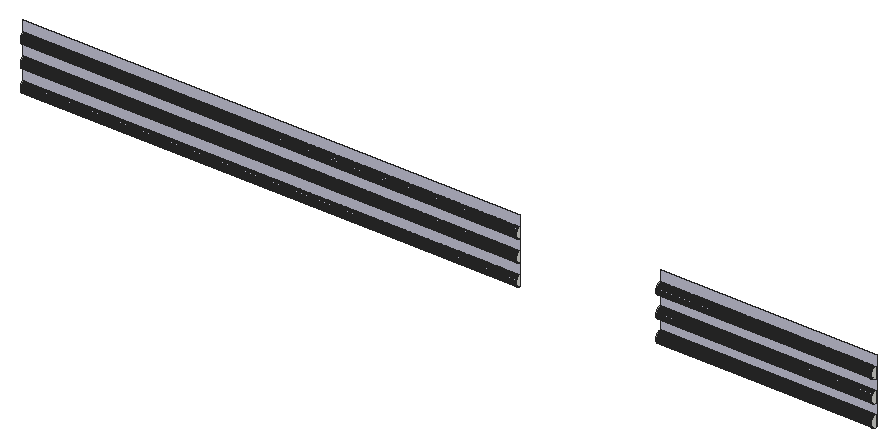
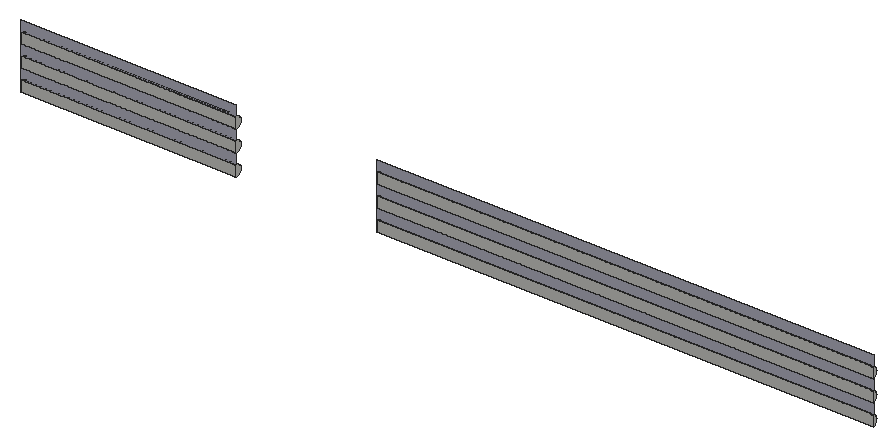
# SketchUp Ruby script. Lengths in millimetres.
U = 1.mm
M = Sketchup.active_model
def pt(a) = Geom::Point3d.new(a.map { |v| v * U })
def face(e, loops, mat)
  f = e.add_face(loops[0].map { |a| pt(a) })
  loops[1..].each { |l| e.add_face(l.map { |a| pt(a) }).erase! }
  f.material = f.back_material = mat if mat
  f
end
# faces: each face lists its corners as indices into pts; further lists are holes
def faces(e, pts, list, mat = nil) = list.each { |f| face(e, (f[0].is_a?(Array) ? f : [f]).map { |l| l.map { |i| pts[i] } }, mat) }
# xy, xz, yz: faces in a plane at the given z, y or x. An outline is a flat list of corners, or four numbers for a rectangle; further outlines are holes
def ring(l) = l.size == 4 ? [[l[0], l[1]], [l[2], l[1]], [l[2], l[3]], [l[0], l[3]]] : l.each_slice(2).to_a
def flat(e, list, mat, &to3) = list.each { |f| face(e, (f[0].is_a?(Array) ? f : [f]).map { |l| ring(l).map { |u, v| to3.(u, v) } }, mat) }
def xy(e, z, list, mat = nil) = flat(e, list, mat) { |x, y| [x, y, z] }
def xz(e, y, list, mat = nil) = flat(e, list, mat) { |x, z| [x, y, z] }
def yz(e, x, list, mat = nil) = flat(e, list, mat) { |y, z| [x, y, z] }
def lines(e, pts, list) = list.each { |a, b| e.add_line(pt(pts[a]), pt(pts[b])) }
# prism: a flat outline (further loops are holes) pulled along v
def prism(e, loops, v, mat = nil)
  f = face(e, loops, mat); d = Geom::Vector3d.new(v.map { |x| x * U })
  f.pushpull(f.normal.samedirection?(d) ? d.length : -d.length)
end
def box(e, o, s, mat = nil) = prism(e, [[o, [o[0] + s[0], o[1], o[2]], [o[0] + s[0], o[1] + s[1], o[2]], [o[0], o[1] + s[1], o[2]]]], [0, 0, s[2]], mat)
def at(x, y, z, deg = 0) = Geom::Transformation.translation(pt([x, y, z])) * Geom::Transformation.rotation(ORIGIN, Z_AXIS, deg.degrees)
def axes(o, x, y, z) = Geom::Transformation.new([*x, 0, *y, 0, *z, 0, *pt(o).to_a, 1])
def part(name) = M.definitions.add(name)
# library, detail: a bought-in or finely detailed component or shape, given as its bounding box
def library(name, o, s) = part(name).tap { |d| box(d.entities, o, s) }
def detail(e, o, s) = box(e.add_group.entities, o, s)
def put(e, d, t, mat = nil) = e.add_instance(d, t).tap { |i| i.material = mat if mat }
def group(e, t, mat = nil) = e.add_group.tap { |g| g.transformation = t; g.material = mat if mat }.entities
root = M.entities
M.materials.add("[0116_Lavender]").color = [197, 197, 214]
xz(root,16548.1,[[11038.5,5045.1,25059.3,5349.9],[29021.7,5045.1,35117.7,5349.9],[11038.5,5654.7,25059.3,5959.5],[29021.7,5654.7,35117.7,5959.5],[11038.5,6264.3,25059.3,6569.1],
  [29021.7,6264.3,35117.7,6569.1]])
xz(root,16548.1,[[11038.5,5349.9,25059.3,5654.7],[29021.7,5349.9,35117.7,5654.7],[11038.5,5959.5,25059.3,6264.3],[29021.7,5959.5,35117.7,6264.3],[11038.5,6569.1,25059.3,6873.9],
  [29021.7,6569.1,35117.7,6873.9]],"[0116_Lavender]")
yz(root,11038.5,[[16548.1,5045.1,16536.2,5050.4,16524.8,5056.7,16514,5063.8,16503.7,5071.8,16494.1,5080.6,16485.2,5090.1,16477.1,5100.2,16469.8,5111,16463.4,5122.3,16458,5134.1,16453.4,5146.3,16449.9,5158.8,16447.3,5171.6,16445.8,5184.5,16445.3,5197.5,16445.8,5210.5,16447.3,5223.4,16449.9,5236.1,16453.4,5248.6,16458,5260.8,16463.4,5272.6,16469.8,5283.9,16477.1,5294.7,16485.2,5304.9,16494.1,5314.4,16503.7,5323.2,16514,5331.1,16524.8,5338.3,16536.2,5344.5,16548.1,5349.9],[16548.1,5654.7,16536.2,5660,16524.8,5666.3,16514,5673.4,16503.7,5681.4,16494.1,5690.2,16485.2,5699.7,16477.1,5709.8,16469.8,5720.6,16463.4,5731.9,16458,5743.7,16453.4,5755.9,16449.9,5768.4,16447.3,5781.2,16445.8,5794.1,16445.3,5807.1,16445.8,5820.1,16447.3,5833,16449.9,5845.7,16453.4,5858.2,16458,5870.4,16463.4,5882.2,16469.8,5893.5,16477.1,5904.3,16485.2,5914.5,16494.1,5924,16503.7,5932.8,16514,5940.7,16524.8,5947.9,16536.2,5954.1,16548.1,5959.5],[16548.1,6264.3,16536.2,6269.6,16524.8,6275.9,16514,6283,16503.7,6291,16494.1,6299.8,16485.2,6309.3,16477.1,6319.4,16469.8,6330.2,16463.4,6341.5,16458,6353.3,16453.4,6365.5,16449.9,6378,16447.3,6390.8,16445.8,6403.7,16445.3,6416.7,16445.8,6429.7,16447.3,6442.6,16449.9,6455.3,16453.4,6467.8,16458,6480,16463.4,6491.8,16469.8,6503.1,16477.1,6513.9,16485.2,6524.1,16494.1,6533.6,16503.7,6542.4,16514,6550.3,16524.8,6557.5,16536.2,6563.7,16548.1,6569.1]])
yz(root,25059.3,[[16548.1,5045.1,16548.1,5349.9,16536.2,5344.5,16524.8,5338.3,16514,5331.1,16503.7,5323.2,16494.1,5314.4,16485.2,5304.9,16477.1,5294.7,16469.8,5283.9,16463.4,5272.6,16458,5260.8,16453.4,5248.6,16449.9,5236.1,16447.3,5223.4,16445.8,5210.5,16445.3,5197.5,16445.8,5184.5,16447.3,5171.6,16449.9,5158.8,16453.4,5146.3,16458,5134.1,16463.4,5122.3,16469.8,5111,16477.1,5100.2,16485.2,5090.1,16494.1,5080.6,16503.7,5071.8,16514,5063.8,16524.8,5056.7,16536.2,5050.4],[16548.1,5654.7,16548.1,5959.5,16536.2,5954.1,16524.8,5947.9,16514,5940.7,16503.7,5932.8,16494.1,5924,16485.2,5914.5,16477.1,5904.3,16469.8,5893.5,16463.4,5882.2,16458,5870.4,16453.4,5858.2,16449.9,5845.7,16447.3,5833,16445.8,5820.1,16445.3,5807.1,16445.8,5794.1,16447.3,5781.2,16449.9,5768.4,16453.4,5755.9,16458,5743.7,16463.4,5731.9,16469.8,5720.6,16477.1,5709.8,16485.2,5699.7,16494.1,5690.2,16503.7,5681.4,16514,5673.4,16524.8,5666.3,16536.2,5660],[16548.1,6264.3,16548.1,6569.1,16536.2,6563.7,16524.8,6557.5,16514,6550.3,16503.7,6542.4,16494.1,6533.6,16485.2,6524.1,16477.1,6513.9,16469.8,6503.1,16463.4,6491.8,16458,6480,16453.4,6467.8,16449.9,6455.3,16447.3,6442.6,16445.8,6429.7,16445.3,6416.7,16445.8,6403.7,16447.3,6390.8,16449.9,6378,16453.4,6365.5,16458,6353.3,16463.4,6341.5,16469.8,6330.2,16477.1,6319.4,16485.2,6309.3,16494.1,6299.8,16503.7,6291,16514,6283,16524.8,6275.9,16536.2,6269.6]])
yz(root,29021.7,[[16548.1,5045.1,16540.1,5045.3,16532.2,5045.9,16524.3,5047,16516.4,5048.4,16508.7,5050.3,16501,5052.5,16493.5,5055.2,16486.1,5058.3,16478.9,5061.7,16471.9,5065.5,16465.1,5069.7,16458.5,5074.2,16452.2,5079,16446.1,5084.2,16440.3,5089.7,16434.8,5095.5,16429.7,5101.6,16424.8,5107.9,16420.3,5114.5,16416.1,5121.3,16412.3,5128.3,16408.9,5135.5,16405.8,5142.9,16403.2,5150.4,16400.9,5158,16399,5165.8,16397.6,5173.6,16396.5,5181.5,16395.9,5189.5,16395.7,5197.5,16395.9,5205.5,16396.5,5213.4,16397.6,5221.3,16399,5229.2,16400.9,5236.9,16403.2,5244.6,16405.8,5252.1,16408.9,5259.5,16412.3,5266.7,16416.1,5273.7,16420.3,5280.5,16424.8,5287.1,16429.7,5293.4,16434.8,5299.5,16440.3,5305.2,16446.1,5310.7,16452.2,5315.9,16458.5,5320.8,16465.1,5325.3,16471.9,5329.5,16478.9,5333.3,16486.1,5336.7,16493.5,5339.8,16501,5342.4,16508.7,5344.7,16516.4,5346.5,16524.3,5348,16532.2,5349,16540.1,5349.7,16548.1,5349.9],[16548.1,5654.7,16540.1,5654.9,16532.2,5655.5,16524.3,5656.6,16516.4,5658,16508.7,5659.9,16501,5662.1,16493.5,5664.8,16486.1,5667.9,16478.9,5671.3,16471.9,5675.1,16465.1,5679.3,16458.5,5683.8,16452.2,5688.6,16446.1,5693.8,16440.3,5699.3,16434.8,5705.1,16429.7,5711.2,16424.8,5717.5,16420.3,5724.1,16416.1,5730.9,16412.3,5737.9,16408.9,5745.1,16405.8,5752.5,16403.2,5760,16400.9,5767.6,16399,5775.4,16397.6,5783.2,16396.5,5791.1,16395.9,5799.1,16395.7,5807.1,16395.9,5815.1,16396.5,5823,16397.6,5830.9,16399,5838.8,16400.9,5846.5,16403.2,5854.2,16405.8,5861.7,16408.9,5869.1,16412.3,5876.3,16416.1,5883.3,16420.3,5890.1,16424.8,5896.7,16429.7,5903,16434.8,5909.1,16440.3,5914.8,16446.1,5920.3,16452.2,5925.5,16458.5,5930.4,16465.1,5934.9,16471.9,5939.1,16478.9,5942.9,16486.1,5946.3,16493.5,5949.4,16501,5952,16508.7,5954.3,16516.4,5956.1,16524.3,5957.6,16532.2,5958.6,16540.1,5959.3,16548.1,5959.5],[16548.1,6264.3,16540.1,6264.5,16532.2,6265.1,16524.3,6266.2,16516.4,6267.6,16508.7,6269.5,16501,6271.7,16493.5,6274.4,16486.1,6277.5,16478.9,6280.9,16471.9,6284.7,16465.1,6288.9,16458.5,6293.4,16452.2,6298.2,16446.1,6303.4,16440.3,6308.9,16434.8,6314.7,16429.7,6320.8,16424.8,6327.1,16420.3,6333.7,16416.1,6340.5,16412.3,6347.5,16408.9,6354.7,16405.8,6362.1,16403.2,6369.6,16400.9,6377.2,16399,6385,16397.6,6392.8,16396.5,6400.7,16395.9,6408.7,16395.7,6416.7,16395.9,6424.7,16396.5,6432.6,16397.6,6440.5,16399,6448.4,16400.9,6456.1,16403.2,6463.8,16405.8,6471.3,16408.9,6478.7,16412.3,6485.9,16416.1,6492.9,16420.3,6499.7,16424.8,6506.3,16429.7,6512.6,16434.8,6518.7,16440.3,6524.4,16446.1,6529.9,16452.2,6535.1,16458.5,6540,16465.1,6544.5,16471.9,6548.7,16478.9,6552.5,16486.1,6555.9,16493.5,6559,16501,6561.6,16508.7,6563.9,16516.4,6565.7,16524.3,6567.2,16532.2,6568.2,16540.1,6568.9,16548.1,6569.1]])
yz(root,35117.7,[[16548.1,5045.1,16548.1,5349.9,16540.1,5349.7,16532.2,5349,16524.3,5348,16516.4,5346.5,16508.7,5344.7,16501,5342.4,16493.5,5339.8,16486.1,5336.7,16478.9,5333.3,16471.9,5329.5,16465.1,5325.3,16458.5,5320.8,16452.2,5315.9,16446.1,5310.7,16440.3,5305.2,16434.8,5299.5,16429.7,5293.4,16424.8,5287.1,16420.3,5280.5,16416.1,5273.7,16412.3,5266.7,16408.9,5259.5,16405.8,5252.1,16403.2,5244.6,16400.9,5236.9,16399,5229.2,16397.6,5221.3,16396.5,5213.4,16395.9,5205.5,16395.7,5197.5,16395.9,5189.5,16396.5,5181.5,16397.6,5173.6,16399,5165.8,16400.9,5158,16403.2,5150.4,16405.8,5142.9,16408.9,5135.5,16412.3,5128.3,16416.1,5121.3,16420.3,5114.5,16424.8,5107.9,16429.7,5101.6,16434.8,5095.5,16440.3,5089.7,16446.1,5084.2,16452.2,5079,16458.5,5074.2,16465.1,5069.7,16471.9,5065.5,16478.9,5061.7,16486.1,5058.3,16493.5,5055.2,16501,5052.5,16508.7,5050.3,16516.4,5048.4,16524.3,5047,16532.2,5045.9,16540.1,5045.3],[16548.1,5654.7,16548.1,5959.5,16540.1,5959.3,16532.2,5958.6,16524.3,5957.6,16516.4,5956.1,16508.7,5954.3,16501,5952,16493.5,5949.4,16486.1,5946.3,16478.9,5942.9,16471.9,5939.1,16465.1,5934.9,16458.5,5930.4,16452.2,5925.5,16446.1,5920.3,16440.3,5914.8,16434.8,5909.1,16429.7,5903,16424.8,5896.7,16420.3,5890.1,16416.1,5883.3,16412.3,5876.3,16408.9,5869.1,16405.8,5861.7,16403.2,5854.2,16400.9,5846.5,16399,5838.8,16397.6,5830.9,16396.5,5823,16395.9,5815.1,16395.7,5807.1,16395.9,5799.1,16396.5,5791.1,16397.6,5783.2,16399,5775.4,16400.9,5767.6,16403.2,5760,16405.8,5752.5,16408.9,5745.1,16412.3,5737.9,16416.1,5730.9,16420.3,5724.1,16424.8,5717.5,16429.7,5711.2,16434.8,5705.1,16440.3,5699.3,16446.1,5693.8,16452.2,5688.6,16458.5,5683.8,16465.1,5679.3,16471.9,5675.1,16478.9,5671.3,16486.1,5667.9,16493.5,5664.8,16501,5662.1,16508.7,5659.9,16516.4,5658,16524.3,5656.6,16532.2,5655.5,16540.1,5654.9],[16548.1,6264.3,16548.1,6569.1,16540.1,6568.9,16532.2,6568.2,16524.3,6567.2,16516.4,6565.7,16508.7,6563.9,16501,6561.6,16493.5,6559,16486.1,6555.9,16478.9,6552.5,16471.9,6548.7,16465.1,6544.5,16458.5,6540,16452.2,6535.1,16446.1,6529.9,16440.3,6524.4,16434.8,6518.7,16429.7,6512.6,16424.8,6506.3,16420.3,6499.7,16416.1,6492.9,16412.3,6485.9,16408.9,6478.7,16405.8,6471.3,16403.2,6463.8,16400.9,6456.1,16399,6448.4,16397.6,6440.5,16396.5,6432.6,16395.9,6424.7,16395.7,6416.7,16395.9,6408.7,16396.5,6400.7,16397.6,6392.8,16399,6385,16400.9,6377.2,16403.2,6369.6,16405.8,6362.1,16408.9,6354.7,16412.3,6347.5,16416.1,6340.5,16420.3,6333.7,16424.8,6327.1,16429.7,6320.8,16434.8,6314.7,16440.3,6308.9,16446.1,6303.4,16452.2,6298.2,16458.5,6293.4,16465.1,6288.9,16471.9,6284.7,16478.9,6280.9,16486.1,6277.5,16493.5,6274.4,16501,6271.7,16508.7,6269.5,16516.4,6267.6,16524.3,6266.2,16532.2,6265.1,16540.1,6264.5]])
p = [[25059.3,16548.1,5045.1],[25059.3,16536.2,5050.4],[11038.5,16536.2,5050.4],[11038.5,16548.1,5045.1],[35117.7,16548.1,5045.1],[35117.7,16540.1,5045.3],
  [29021.7,16540.1,5045.3],[29021.7,16548.1,5045.1],[35117.7,16532.2,5045.9],[29021.7,16532.2,5045.9],[35117.7,16524.3,5047],[29021.7,16524.3,5047],
  [35117.7,16516.4,5048.4],[29021.7,16516.4,5048.4],[35117.7,16508.7,5050.3],[29021.7,16508.7,5050.3],[35117.7,16501,5052.5],[29021.7,16501,5052.5],
  [25059.3,16524.8,5056.7],[11038.5,16524.8,5056.7],[35117.7,16493.5,5055.2],[29021.7,16493.5,5055.2],[35117.7,16486.1,5058.3],[29021.7,16486.1,5058.3],
  [25059.3,16514,5063.8],[11038.5,16514,5063.8],[35117.7,16478.9,5061.7],[29021.7,16478.9,5061.7],[35117.7,16471.9,5065.5],[29021.7,16471.9,5065.5],
  [25059.3,16503.7,5071.8],[11038.5,16503.7,5071.8],[35117.7,16465.1,5069.7],[29021.7,16465.1,5069.7],[35117.7,16458.5,5074.2],[29021.7,16458.5,5074.2],
  [25059.3,16494.1,5080.6],[11038.5,16494.1,5080.6],[35117.7,16452.2,5079],[29021.7,16452.2,5079],[35117.7,16446.1,5084.2],[29021.7,16446.1,5084.2],
  [25059.3,16485.2,5090.1],[11038.5,16485.2,5090.1],[35117.7,16440.3,5089.7],[29021.7,16440.3,5089.7],[35117.7,16434.8,5095.5],[29021.7,16434.8,5095.5],
  [25059.3,16477.1,5100.2],[11038.5,16477.1,5100.2],[35117.7,16429.7,5101.6],[29021.7,16429.7,5101.6],[25059.3,16469.8,5111],[11038.5,16469.8,5111],
  [35117.7,16424.8,5107.9],[29021.7,16424.8,5107.9],[35117.7,16420.3,5114.5],[29021.7,16420.3,5114.5],[25059.3,16463.4,5122.3],[11038.5,16463.4,5122.3],
  [35117.7,16416.1,5121.3],[29021.7,16416.1,5121.3],[35117.7,16412.3,5128.3],[29021.7,16412.3,5128.3],[25059.3,16458,5134.1],[11038.5,16458,5134.1],
  [35117.7,16408.9,5135.5],[29021.7,16408.9,5135.5],[25059.3,16453.4,5146.3],[11038.5,16453.4,5146.3],[35117.7,16405.8,5142.9],[29021.7,16405.8,5142.9],
  [35117.7,16403.2,5150.4],[29021.7,16403.2,5150.4],[25059.3,16449.9,5158.8],[11038.5,16449.9,5158.8],[35117.7,16400.9,5158],[29021.7,16400.9,5158],
  [35117.7,16399,5165.8],[29021.7,16399,5165.8],[25059.3,16447.3,5171.6],[11038.5,16447.3,5171.6],[35117.7,16397.6,5173.6],[29021.7,16397.6,5173.6],
  [25059.3,16445.8,5184.5],[11038.5,16445.8,5184.5],[35117.7,16396.5,5181.5],[29021.7,16396.5,5181.5],[35117.7,16395.9,5189.5],[29021.7,16395.9,5189.5],
  [25059.3,16445.3,5197.5],[11038.5,16445.3,5197.5],[35117.7,16395.7,5197.5],[29021.7,16395.7,5197.5],[35117.7,16395.9,5205.5],[29021.7,16395.9,5205.5],
  [25059.3,16445.8,5210.5],[11038.5,16445.8,5210.5],[35117.7,16396.5,5213.4],[29021.7,16396.5,5213.4],[25059.3,16447.3,5223.4],[11038.5,16447.3,5223.4],
  [35117.7,16397.6,5221.3],[29021.7,16397.6,5221.3],[35117.7,16399,5229.2],[29021.7,16399,5229.2],[25059.3,16449.9,5236.1],[11038.5,16449.9,5236.1],
  [35117.7,16400.9,5236.9],[29021.7,16400.9,5236.9],[25059.3,16453.4,5248.6],[11038.5,16453.4,5248.6],[35117.7,16403.2,5244.6],[29021.7,16403.2,5244.6],
  [35117.7,16405.8,5252.1],[29021.7,16405.8,5252.1],[25059.3,16458,5260.8],[11038.5,16458,5260.8],[35117.7,16408.9,5259.5],[29021.7,16408.9,5259.5],
  [35117.7,16412.3,5266.7],[29021.7,16412.3,5266.7],[25059.3,16463.4,5272.6],[11038.5,16463.4,5272.6],[35117.7,16416.1,5273.7],[29021.7,16416.1,5273.7],
  [25059.3,16469.8,5283.9],[11038.5,16469.8,5283.9],[35117.7,16420.3,5280.5],[29021.7,16420.3,5280.5],[35117.7,16424.8,5287.1],[29021.7,16424.8,5287.1],
  [25059.3,16477.1,5294.7],[11038.5,16477.1,5294.7],[35117.7,16429.7,5293.4],[29021.7,16429.7,5293.4],[35117.7,16434.8,5299.5],[29021.7,16434.8,5299.5],
  [25059.3,16485.2,5304.9],[11038.5,16485.2,5304.9],[35117.7,16440.3,5305.2],[29021.7,16440.3,5305.2],[25059.3,16494.1,5314.4],[11038.5,16494.1,5314.4],
  [35117.7,16446.1,5310.7],[29021.7,16446.1,5310.7],[35117.7,16452.2,5315.9],[29021.7,16452.2,5315.9],[25059.3,16503.7,5323.2],[11038.5,16503.7,5323.2],
  [35117.7,16458.5,5320.8],[29021.7,16458.5,5320.8],[35117.7,16465.1,5325.3],[29021.7,16465.1,5325.3],[25059.3,16514,5331.1],[11038.5,16514,5331.1],
  [35117.7,16471.9,5329.5],[29021.7,16471.9,5329.5],[35117.7,16478.9,5333.3],[29021.7,16478.9,5333.3],[25059.3,16524.8,5338.3],[11038.5,16524.8,5338.3],
  [35117.7,16486.1,5336.7],[29021.7,16486.1,5336.7],[35117.7,16493.5,5339.8],[29021.7,16493.5,5339.8],[25059.3,16536.2,5344.5],[11038.5,16536.2,5344.5],
  [35117.7,16501,5342.4],[29021.7,16501,5342.4],[35117.7,16508.7,5344.7],[29021.7,16508.7,5344.7],[25059.3,16548.1,5349.9],[11038.5,16548.1,5349.9],
  [35117.7,16516.4,5346.5],[29021.7,16516.4,5346.5],[35117.7,16524.3,5348],[29021.7,16524.3,5348],[35117.7,16532.2,5349],[29021.7,16532.2,5349],
  [35117.7,16540.1,5349.7],[29021.7,16540.1,5349.7],[35117.7,16548.1,5349.9],[29021.7,16548.1,5349.9],[25059.3,16548.1,5654.7],[25059.3,16536.2,5660],
  [11038.5,16536.2,5660],[11038.5,16548.1,5654.7],[35117.7,16548.1,5654.7],[35117.7,16540.1,5654.9],[29021.7,16540.1,5654.9],[29021.7,16548.1,5654.7],
  [35117.7,16532.2,5655.5],[29021.7,16532.2,5655.5],[35117.7,16524.3,5656.6],[29021.7,16524.3,5656.6],[35117.7,16516.4,5658],[29021.7,16516.4,5658],
  [35117.7,16508.7,5659.9],[29021.7,16508.7,5659.9],[35117.7,16501,5662.1],[29021.7,16501,5662.1],[25059.3,16524.8,5666.3],[11038.5,16524.8,5666.3],
  [35117.7,16493.5,5664.8],[29021.7,16493.5,5664.8],[35117.7,16486.1,5667.9],[29021.7,16486.1,5667.9],[25059.3,16514,5673.4],[11038.5,16514,5673.4],
  [35117.7,16478.9,5671.3],[29021.7,16478.9,5671.3],[35117.7,16471.9,5675.1],[29021.7,16471.9,5675.1],[25059.3,16503.7,5681.4],[11038.5,16503.7,5681.4],
  [35117.7,16465.1,5679.3],[29021.7,16465.1,5679.3],[35117.7,16458.5,5683.8],[29021.7,16458.5,5683.8],[25059.3,16494.1,5690.2],[11038.5,16494.1,5690.2],
  [35117.7,16452.2,5688.6],[29021.7,16452.2,5688.6],[35117.7,16446.1,5693.8],[29021.7,16446.1,5693.8],[25059.3,16485.2,5699.7],[11038.5,16485.2,5699.7],
  [35117.7,16440.3,5699.3],[29021.7,16440.3,5699.3],[35117.7,16434.8,5705.1],[29021.7,16434.8,5705.1],[25059.3,16477.1,5709.8],[11038.5,16477.1,5709.8],
  [35117.7,16429.7,5711.2],[29021.7,16429.7,5711.2],[25059.3,16469.8,5720.6],[11038.5,16469.8,5720.6],[35117.7,16424.8,5717.5],[29021.7,16424.8,5717.5],
  [35117.7,16420.3,5724.1],[29021.7,16420.3,5724.1],[25059.3,16463.4,5731.9],[11038.5,16463.4,5731.9],[35117.7,16416.1,5730.9],[29021.7,16416.1,5730.9],
  [35117.7,16412.3,5737.9],[29021.7,16412.3,5737.9],[25059.3,16458,5743.7],[11038.5,16458,5743.7],[35117.7,16408.9,5745.1],[29021.7,16408.9,5745.1],
  [25059.3,16453.4,5755.9],[11038.5,16453.4,5755.9],[35117.7,16405.8,5752.5],[29021.7,16405.8,5752.5],[35117.7,16403.2,5760],[29021.7,16403.2,5760],
  [25059.3,16449.9,5768.4],[11038.5,16449.9,5768.4],[35117.7,16400.9,5767.6],[29021.7,16400.9,5767.6],[35117.7,16399,5775.4],[29021.7,16399,5775.4],
  [25059.3,16447.3,5781.2],[11038.5,16447.3,5781.2],[35117.7,16397.6,5783.2],[29021.7,16397.6,5783.2],[25059.3,16445.8,5794.1],[11038.5,16445.8,5794.1],
  [35117.7,16396.5,5791.1],[29021.7,16396.5,5791.1],[35117.7,16395.9,5799.1],[29021.7,16395.9,5799.1],[25059.3,16445.3,5807.1],[11038.5,16445.3,5807.1],
  [35117.7,16395.7,5807.1],[29021.7,16395.7,5807.1],[35117.7,16395.9,5815.1],[29021.7,16395.9,5815.1],[25059.3,16445.8,5820.1],[11038.5,16445.8,5820.1],
  [35117.7,16396.5,5823],[29021.7,16396.5,5823],[25059.3,16447.3,5833],[11038.5,16447.3,5833],[35117.7,16397.6,5830.9],[29021.7,16397.6,5830.9],
  [35117.7,16399,5838.8],[29021.7,16399,5838.8],[25059.3,16449.9,5845.7],[11038.5,16449.9,5845.7],[35117.7,16400.9,5846.5],[29021.7,16400.9,5846.5],
  [25059.3,16453.4,5858.2],[11038.5,16453.4,5858.2],[35117.7,16403.2,5854.2],[29021.7,16403.2,5854.2],[35117.7,16405.8,5861.7],[29021.7,16405.8,5861.7],
  [25059.3,16458,5870.4],[11038.5,16458,5870.4],[35117.7,16408.9,5869.1],[29021.7,16408.9,5869.1],[35117.7,16412.3,5876.3],[29021.7,16412.3,5876.3],
  [25059.3,16463.4,5882.2],[11038.5,16463.4,5882.2],[35117.7,16416.1,5883.3],[29021.7,16416.1,5883.3],[25059.3,16469.8,5893.5],[11038.5,16469.8,5893.5],
  [35117.7,16420.3,5890.1],[29021.7,16420.3,5890.1],[35117.7,16424.8,5896.7],[29021.7,16424.8,5896.7],[25059.3,16477.1,5904.3],[11038.5,16477.1,5904.3],
  [35117.7,16429.7,5903],[29021.7,16429.7,5903],[35117.7,16434.8,5909.1],[29021.7,16434.8,5909.1],[25059.3,16485.2,5914.5],[11038.5,16485.2,5914.5],
  [35117.7,16440.3,5914.8],[29021.7,16440.3,5914.8],[25059.3,16494.1,5924],[11038.5,16494.1,5924],[35117.7,16446.1,5920.3],[29021.7,16446.1,5920.3],
  [35117.7,16452.2,5925.5],[29021.7,16452.2,5925.5],[25059.3,16503.7,5932.8],[11038.5,16503.7,5932.8],[35117.7,16458.5,5930.4],[29021.7,16458.5,5930.4],
  [35117.7,16465.1,5934.9],[29021.7,16465.1,5934.9],[25059.3,16514,5940.7],[11038.5,16514,5940.7],[35117.7,16471.9,5939.1],[29021.7,16471.9,5939.1],
  [35117.7,16478.9,5942.9],[29021.7,16478.9,5942.9],[25059.3,16524.8,5947.9],[11038.5,16524.8,5947.9],[35117.7,16486.1,5946.3],[29021.7,16486.1,5946.3],
  [35117.7,16493.5,5949.4],[29021.7,16493.5,5949.4],[25059.3,16536.2,5954.1],[11038.5,16536.2,5954.1],[35117.7,16501,5952],[29021.7,16501,5952],
  [35117.7,16508.7,5954.3],[29021.7,16508.7,5954.3],[25059.3,16548.1,5959.5],[11038.5,16548.1,5959.5],[35117.7,16516.4,5956.1],[29021.7,16516.4,5956.1],
  [35117.7,16524.3,5957.6],[29021.7,16524.3,5957.6],[35117.7,16532.2,5958.6],[29021.7,16532.2,5958.6],[35117.7,16540.1,5959.3],[29021.7,16540.1,5959.3],
  [35117.7,16548.1,5959.5],[29021.7,16548.1,5959.5],[25059.3,16548.1,6264.3],[25059.3,16536.2,6269.6],[11038.5,16536.2,6269.6],[11038.5,16548.1,6264.3],
  [35117.7,16548.1,6264.3],[35117.7,16540.1,6264.5],[29021.7,16540.1,6264.5],[29021.7,16548.1,6264.3],[35117.7,16532.2,6265.1],[29021.7,16532.2,6265.1],
  [35117.7,16524.3,6266.2],[29021.7,16524.3,6266.2],[35117.7,16516.4,6267.6],[29021.7,16516.4,6267.6],[35117.7,16508.7,6269.5],[29021.7,16508.7,6269.5],
  [35117.7,16501,6271.7],[29021.7,16501,6271.7],[25059.3,16524.8,6275.9],[11038.5,16524.8,6275.9],[35117.7,16493.5,6274.4],[29021.7,16493.5,6274.4],
  [35117.7,16486.1,6277.5],[29021.7,16486.1,6277.5],[25059.3,16514,6283],[11038.5,16514,6283],[35117.7,16478.9,6280.9],[29021.7,16478.9,6280.9],
  [35117.7,16471.9,6284.7],[29021.7,16471.9,6284.7],[25059.3,16503.7,6291],[11038.5,16503.7,6291],[35117.7,16465.1,6288.9],[29021.7,16465.1,6288.9],
  [35117.7,16458.5,6293.4],[29021.7,16458.5,6293.4],[25059.3,16494.1,6299.8],[11038.5,16494.1,6299.8],[35117.7,16452.2,6298.2],[29021.7,16452.2,6298.2],
  [35117.7,16446.1,6303.4],[29021.7,16446.1,6303.4],[25059.3,16485.2,6309.3],[11038.5,16485.2,6309.3],[35117.7,16440.3,6308.9],[29021.7,16440.3,6308.9],
  [35117.7,16434.8,6314.7],[29021.7,16434.8,6314.7],[25059.3,16477.1,6319.4],[11038.5,16477.1,6319.4],[35117.7,16429.7,6320.8],[29021.7,16429.7,6320.8],
  [25059.3,16469.8,6330.2],[11038.5,16469.8,6330.2],[35117.7,16424.8,6327.1],[29021.7,16424.8,6327.1],[35117.7,16420.3,6333.7],[29021.7,16420.3,6333.7],
  [25059.3,16463.4,6341.5],[11038.5,16463.4,6341.5],[35117.7,16416.1,6340.5],[29021.7,16416.1,6340.5],[35117.7,16412.3,6347.5],[29021.7,16412.3,6347.5],
  [25059.3,16458,6353.3],[11038.5,16458,6353.3],[35117.7,16408.9,6354.7],[29021.7,16408.9,6354.7],[25059.3,16453.4,6365.5],[11038.5,16453.4,6365.5],
  [35117.7,16405.8,6362.1],[29021.7,16405.8,6362.1],[35117.7,16403.2,6369.6],[29021.7,16403.2,6369.6],[25059.3,16449.9,6378],[11038.5,16449.9,6378],
  [35117.7,16400.9,6377.2],[29021.7,16400.9,6377.2],[35117.7,16399,6385],[29021.7,16399,6385],[25059.3,16447.3,6390.8],[11038.5,16447.3,6390.8],
  [35117.7,16397.6,6392.8],[29021.7,16397.6,6392.8],[25059.3,16445.8,6403.7],[11038.5,16445.8,6403.7],[35117.7,16396.5,6400.7],[29021.7,16396.5,6400.7],
  [35117.7,16395.9,6408.7],[29021.7,16395.9,6408.7],[25059.3,16445.3,6416.7],[11038.5,16445.3,6416.7],[35117.7,16395.7,6416.7],[29021.7,16395.7,6416.7],
  [35117.7,16395.9,6424.7],[29021.7,16395.9,6424.7],[25059.3,16445.8,6429.7],[11038.5,16445.8,6429.7],[35117.7,16396.5,6432.6],[29021.7,16396.5,6432.6],
  [25059.3,16447.3,6442.6],[11038.5,16447.3,6442.6],[35117.7,16397.6,6440.5],[29021.7,16397.6,6440.5],[35117.7,16399,6448.4],[29021.7,16399,6448.4],
  [25059.3,16449.9,6455.3],[11038.5,16449.9,6455.3],[35117.7,16400.9,6456.1],[29021.7,16400.9,6456.1],[25059.3,16453.4,6467.8],[11038.5,16453.4,6467.8],
  [35117.7,16403.2,6463.8],[29021.7,16403.2,6463.8],[35117.7,16405.8,6471.3],[29021.7,16405.8,6471.3],[25059.3,16458,6480],[11038.5,16458,6480],
  [35117.7,16408.9,6478.7],[29021.7,16408.9,6478.7],[35117.7,16412.3,6485.9],[29021.7,16412.3,6485.9],[25059.3,16463.4,6491.8],[11038.5,16463.4,6491.8],
  [35117.7,16416.1,6492.9],[29021.7,16416.1,6492.9],[25059.3,16469.8,6503.1],[11038.5,16469.8,6503.1],[35117.7,16420.3,6499.7],[29021.7,16420.3,6499.7],
  [35117.7,16424.8,6506.3],[29021.7,16424.8,6506.3],[25059.3,16477.1,6513.9],[11038.5,16477.1,6513.9],[35117.7,16429.7,6512.6],[29021.7,16429.7,6512.6],
  [35117.7,16434.8,6518.7],[29021.7,16434.8,6518.7],[25059.3,16485.2,6524.1],[11038.5,16485.2,6524.1],[35117.7,16440.3,6524.4],[29021.7,16440.3,6524.4],
  [25059.3,16494.1,6533.6],[11038.5,16494.1,6533.6],[35117.7,16446.1,6529.9],[29021.7,16446.1,6529.9],[35117.7,16452.2,6535.1],[29021.7,16452.2,6535.1],
  [25059.3,16503.7,6542.4],[11038.5,16503.7,6542.4],[35117.7,16458.5,6540],[29021.7,16458.5,6540],[35117.7,16465.1,6544.5],[29021.7,16465.1,6544.5],
  [25059.3,16514,6550.3],[11038.5,16514,6550.3],[35117.7,16471.9,6548.7],[29021.7,16471.9,6548.7],[35117.7,16478.9,6552.5],[29021.7,16478.9,6552.5],
  [25059.3,16524.8,6557.5],[11038.5,16524.8,6557.5],[35117.7,16486.1,6555.9],[29021.7,16486.1,6555.9],[35117.7,16493.5,6559],[29021.7,16493.5,6559],
  [25059.3,16536.2,6563.7],[11038.5,16536.2,6563.7],[35117.7,16501,6561.6],[29021.7,16501,6561.6],[35117.7,16508.7,6563.9],[29021.7,16508.7,6563.9],
  [25059.3,16548.1,6569.1],[11038.5,16548.1,6569.1],[35117.7,16516.4,6565.7],[29021.7,16516.4,6565.7],[35117.7,16524.3,6567.2],[29021.7,16524.3,6567.2],
  [35117.7,16532.2,6568.2],[29021.7,16532.2,6568.2],[35117.7,16540.1,6568.9],[29021.7,16540.1,6568.9],[35117.7,16548.1,6569.1],[29021.7,16548.1,6569.1]]
faces(root,p,[[0,1,2,3],[4,5,6,7],[5,8,9,6],[8,10,11,9],[10,12,13,11],[12,14,15,13],[14,16,17,15],[1,18,19,2],
  [16,20,21,17],[20,22,23,21],[18,24,25,19],[22,26,27,23],[26,28,29,27],[24,30,31,25],[28,32,33,29],[32,34,35,33],
  [30,36,37,31],[34,38,39,35],[38,40,41,39],[36,42,43,37],[40,44,45,41],[44,46,47,45],[42,48,49,43],[46,50,51,47],
  [48,52,53,49],[50,54,55,51],[54,56,57,55],[52,58,59,53],[56,60,61,57],[60,62,63,61],[58,64,65,59],[62,66,67,63],
  [64,68,69,65],[66,70,71,67],[70,72,73,71],[68,74,75,69],[72,76,77,73],[76,78,79,77],[74,80,81,75],[78,82,83,79],
  [80,84,85,81],[82,86,87,83],[86,88,89,87],[84,90,91,85],[88,92,93,89],[92,94,95,93],[90,96,97,91],[94,98,99,95],
  [96,100,101,97],[98,102,103,99],[102,104,105,103],[100,106,107,101],[104,108,109,105],[106,110,111,107],[108,112,113,109],[112,114,115,113],
  [110,116,117,111],[114,118,119,115],[118,120,121,119],[116,122,123,117],[120,124,125,121],[122,126,127,123],[124,128,129,125],[128,130,131,129],
  [126,132,133,127],[130,134,135,131],[134,136,137,135],[132,138,139,133],[136,140,141,137],[138,142,143,139],[140,144,145,141],[144,146,147,145],
  [142,148,149,143],[146,150,151,147],[150,152,153,151],[148,154,155,149],[152,156,157,153],[156,158,159,157],[154,160,161,155],[158,162,163,159],
  [162,164,165,163],[160,166,167,161],[164,168,169,165],[168,170,171,169],[166,172,173,167],[170,174,175,171],[174,176,177,175],[176,178,179,177],
  [178,180,181,179],[180,182,183,181],[184,185,186,187],[188,189,190,191],[189,192,193,190],[192,194,195,193],[194,196,197,195],[196,198,199,197],
  [198,200,201,199],[185,202,203,186],[200,204,205,201],[204,206,207,205],[202,208,209,203],[206,210,211,207],[210,212,213,211],[208,214,215,209],
  [212,216,217,213],[216,218,219,217],[214,220,221,215],[218,222,223,219],[222,224,225,223],[220,226,227,221],[224,228,229,225],[228,230,231,229],
  [226,232,233,227],[230,234,235,231],[232,236,237,233],[234,238,239,235],[238,240,241,239],[236,242,243,237],[240,244,245,241],[244,246,247,245],
  [242,248,249,243],[246,250,251,247],[248,252,253,249],[250,254,255,251],[254,256,257,255],[252,258,259,253],[256,260,261,257],[260,262,263,261],
  [258,264,265,259],[262,266,267,263],[264,268,269,265],[266,270,271,267],[270,272,273,271],[268,274,275,269],[272,276,277,273],[276,278,279,277],
  [274,280,281,275],[278,282,283,279],[280,284,285,281],[282,286,287,283],[286,288,289,287],[284,290,291,285],[288,292,293,289],[290,294,295,291],
  [292,296,297,293],[296,298,299,297],[294,300,301,295],[298,302,303,299],[302,304,305,303],[300,306,307,301],[304,308,309,305],[306,310,311,307],
  [308,312,313,309],[312,314,315,313],[310,316,317,311],[314,318,319,315],[318,320,321,319],[316,322,323,317],[320,324,325,321],[322,326,327,323],
  [324,328,329,325],[328,330,331,329],[326,332,333,327],[330,334,335,331],[334,336,337,335],[332,338,339,333],[336,340,341,337],[340,342,343,341],
  [338,344,345,339],[342,346,347,343],[346,348,349,347],[344,350,351,345],[348,352,353,349],[352,354,355,353],[350,356,357,351],[354,358,359,355],
  [358,360,361,359],[360,362,363,361],[362,364,365,363],[364,366,367,365],[368,369,370,371],[372,373,374,375],[373,376,377,374],[376,378,379,377],
  [378,380,381,379],[380,382,383,381],[382,384,385,383],[369,386,387,370],[384,388,389,385],[388,390,391,389],[386,392,393,387],[390,394,395,391],
  [394,396,397,395],[392,398,399,393],[396,400,401,397],[400,402,403,401],[398,404,405,399],[402,406,407,403],[406,408,409,407],[404,410,411,405],
  [408,412,413,409],[412,414,415,413],[410,416,417,411],[414,418,419,415],[416,420,421,417],[418,422,423,419],[422,424,425,423],[420,426,427,421],
  [424,428,429,425],[428,430,431,429],[426,432,433,427],[430,434,435,431],[432,436,437,433],[434,438,439,435],[438,440,441,439],[436,442,443,437],
  [440,444,445,441],[444,446,447,445],[442,448,449,443],[446,450,451,447],[448,452,453,449],[450,454,455,451],[454,456,457,455],[452,458,459,453],
  [456,460,461,457],[460,462,463,461],[458,464,465,459],[462,466,467,463],[464,468,469,465],[466,470,471,467],[470,472,473,471],[468,474,475,469],
  [472,476,477,473],[474,478,479,475],[476,480,481,477],[480,482,483,481],[478,484,485,479],[482,486,487,483],[486,488,489,487],[484,490,491,485],
  [488,492,493,489],[490,494,495,491],[492,496,497,493],[496,498,499,497],[494,500,501,495],[498,502,503,499],[502,504,505,503],[500,506,507,501],
  [504,508,509,505],[506,510,511,507],[508,512,513,509],[512,514,515,513],[510,516,517,511],[514,518,519,515],[518,520,521,519],[516,522,523,517],
  [520,524,525,521],[524,526,527,525],[522,528,529,523],[526,530,531,527],[530,532,533,531],[528,534,535,529],[532,536,537,533],[536,538,539,537],
  [534,540,541,535],[538,542,543,539],[542,544,545,543],[544,546,547,545],[546,548,549,547],[548,550,551,549]],"[0116_Lavender]")
